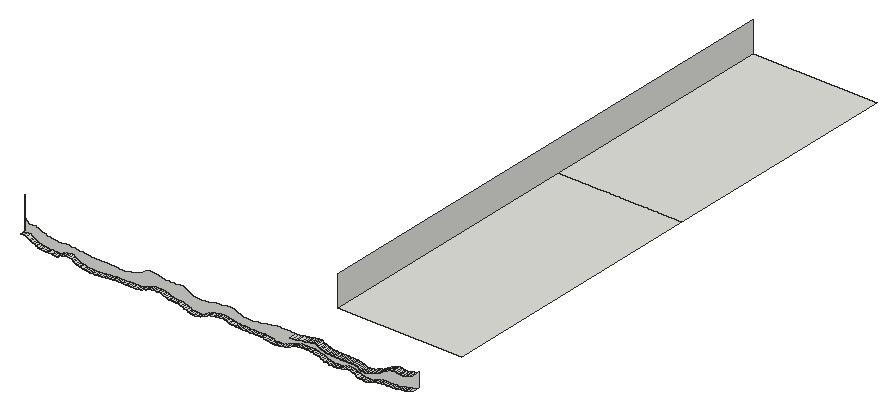
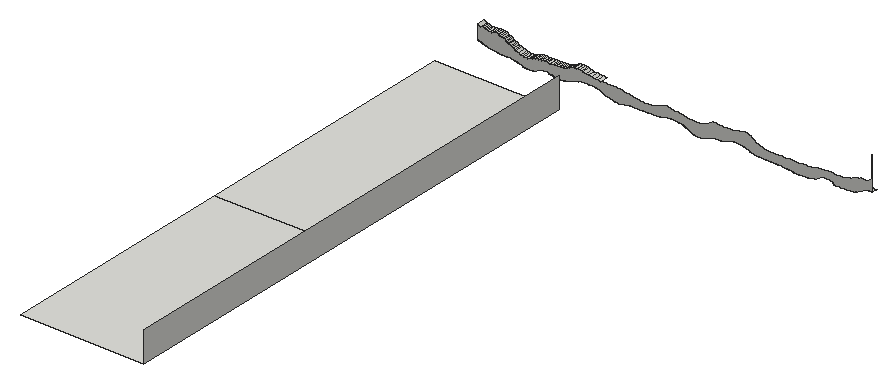
# SketchUp Ruby script. Lengths in inches.
U = 1.inch
M = Sketchup.active_model
def pt(a) = Geom::Point3d.new(a.map { |v| v * U })
def face(e, loops, mat)
  f = e.add_face(loops[0].map { |a| pt(a) })
  loops[1..].each { |l| e.add_face(l.map { |a| pt(a) }).erase! }
  f.material = f.back_material = mat if mat
  f
end
# faces: each face lists its corners as indices into pts; further lists are holes
def faces(e, pts, list, mat = nil) = list.each { |f| face(e, (f[0].is_a?(Array) ? f : [f]).map { |l| l.map { |i| pts[i] } }, mat) }
# xy, xz, yz: faces in a plane at the given z, y or x. An outline is a flat list of corners, or four numbers for a rectangle; further outlines are holes
def ring(l) = l.size == 4 ? [[l[0], l[1]], [l[2], l[1]], [l[2], l[3]], [l[0], l[3]]] : l.each_slice(2).to_a
def flat(e, list, mat, &to3) = list.each { |f| face(e, (f[0].is_a?(Array) ? f : [f]).map { |l| ring(l).map { |u, v| to3.(u, v) } }, mat) }
def xy(e, z, list, mat = nil) = flat(e, list, mat) { |x, y| [x, y, z] }
def xz(e, y, list, mat = nil) = flat(e, list, mat) { |x, z| [x, y, z] }
def yz(e, x, list, mat = nil) = flat(e, list, mat) { |y, z| [x, y, z] }
def lines(e, pts, list) = list.each { |a, b| e.add_line(pt(pts[a]), pt(pts[b])) }
# prism: a flat outline (further loops are holes) pulled along v
def prism(e, loops, v, mat = nil)
  f = face(e, loops, mat); d = Geom::Vector3d.new(v.map { |x| x * U })
  f.pushpull(f.normal.samedirection?(d) ? d.length : -d.length)
end
def box(e, o, s, mat = nil) = prism(e, [[o, [o[0] + s[0], o[1], o[2]], [o[0] + s[0], o[1] + s[1], o[2]], [o[0], o[1] + s[1], o[2]]]], [0, 0, s[2]], mat)
def at(x, y, z, deg = 0) = Geom::Transformation.translation(pt([x, y, z])) * Geom::Transformation.rotation(ORIGIN, Z_AXIS, deg.degrees)
def axes(o, x, y, z) = Geom::Transformation.new([*x, 0, *y, 0, *z, 0, *pt(o).to_a, 1])
def part(name) = M.definitions.add(name)
# library, detail: a bought-in or finely detailed component or shape, given as its bounding box
def library(name, o, s) = part(name).tap { |d| box(d.entities, o, s) }
def detail(e, o, s) = box(e.add_group.entities, o, s)
def put(e, d, t, mat = nil) = e.add_instance(d, t).tap { |i| i.material = mat if mat }
def group(e, t, mat = nil) = e.add_group.tap { |g| g.transformation = t; g.material = mat if mat }.entities
root = M.entities
xy(root,237.65,[[2918.33,566.68,2919.02,568.68],[2919.02,566.68,2919.64,568.68]])
xy(root,238.18,[[3012.28,566.68,3012.96,568.68]])
xy(root,238.33,[[2927.43,566.68,2927.98,568.68],[2927.98,566.68,2928.66,568.68]])
xy(root,238.34,[[2929.34,566.68,2930.27,568.68],[2930.27,566.68,2930.76,568.68],[2930.76,566.68,2931.52,568.68],[2931.52,566.68,2932.15,568.68],[2932.15,566.68,2932.9,568.68],
  [2932.9,566.68,2933.52,568.68],[2933.52,566.68,2934.29,568.68],[2934.29,566.68,2934.91,568.68]])
xy(root,238.62,[[2978.81,566.68,2979.58,568.68],[2979.58,566.68,2980.21,568.68],[2980.21,566.68,2980.97,568.68],[2980.97,566.68,2981.59,568.68],[2981.59,566.68,2982.44,568.68],
  [2982.44,566.68,2983.08,568.68],[2983.08,566.68,2983.7,568.68]])
xy(root,238.625,[[2977.39,566.68,2978.25,568.68]])
xy(root,238.89,[[3033.2,566.68,3033.88,568.68]])
xy(root,238.9,[[3034.64,566.68,3035.26,568.68],[3035.26,566.68,3036.03,568.68]])
xy(root,240.43,[[3001.48,566.68,3002.05,568.68]])
xy(root,241.52,[[2889.03,566.68,2889.09,568.68]])
xy(root,242.28,[[3019.3,565.74,3019.8125,568.68]])
xy(root,242.3,[[3017.54,565.74,3018.21,568.68]])
xy(root,242.33,[[3015.13,565.74,3015.71,568.68]])
xy(root,242.625,[[2994.64,589.83,3043.1,697.21],[2994.64,697.21,3043.1,792.52]])
xz(root,568.68,[[2957.95,236.98,2957.34,237.01,2956.65,237.04,2955.89,237.11,2955.2,237.2,2954.67,237.33,2954,237.68,2953.0625,237.96,2952.5,238.28,2951.72,238.43,2950.94,238.78,2950.27,238.79,2949.73,238.8,2948.97,238.83,2948.22,238.875,2947.65,238.94,2947.07,239.04,2946.41,239.29,2945.83,239.53,2945.3,239.7,2944.61,239.92,2943.98,240.11,2943.2,240.27,2942.58,240.25,2941.875,240.23,2941.11,240.19,2940.4375,240.12,2939.78,240.03,2939.14,239.85,2938.59,239.52,2938.03,239.35,2937.44,239.18,2936.93,238.86,2936.24,238.72,2935.42,238.59,2934.91,238.34,2929.34,238.34,2928.66,238.33,2927.43,238.33,2926.71,238.32,2925.86,238.3,2925.23,238.28,2924.48,238.26,2923.85,238.15,2923.09,238.13,2922.54,238.1,2921.6875,237.98,2921.07,237.94,2920.31,237.89,2919.64,237.65,2918.33,237.65,2917.64,237.66,2916.89,237.67,2916.29,237.68,2915.68,237.71,2914.97,237.76,2914.28,237.82,2913.62,237.9,2912.68,238.21,2912.21,238.31,2911.3,238.43,2910.65,238.74,2910.07,239.11,2909.49,239.38,2909.03,239.71,2908.33,240.11,2907.64,240.09,2906.98,240.05,2906.39,239.99,2905.66,239.88,2905.11,239.69,2904.53,239.55,2903.97,238.9375,2903.44,238.77,2902.7,238.79,2901.83,238.8,2901.32,238.82,2900.28,238.92,2899.59,238.93,2898.89,238.94,2898.19,238.97,2897.51,239.03,2896.82,239.09,2896.04,239.19,2895.53,239.52,2894.97,239.64,2894.52,239.86,2893.73,240.2,2893.13,240.59,2892.59,240.85,2891.57,241.55,2890.3,241.69,2889.09,241.52,2889.09,246.2,2890.66,244.96,2892.05,244.9375,2893.3,244.92,2893.52,244.61,2894.08,244.54,2894.84,244.41,2895.51,244.11,2896.03,243.95,2896.69,243.79,2897.21,243.48,2897.85,243.3,2898.4375,243.14,2898.92,243.06,2899.64,242.85,2900.22,242.78,2901.03,242.73,2901.57,242.68,2902.24,242.51,2902.76,242.46,2903.3,242.58,2903.93,242.57,2904.56,242.81,2905.13,242.86,2905.69,242.89,2906.33,242.92,2906.76,242.625,2907.37,242.65,2907.92,242.62,2908.55,242.58,2909.11,242.57,2909.75,242.48,2910.41,242.38,2911.07,242.34,2911.74,242.24,2912.91,241.96,2913.68,241.89,2914.5,241.83,2915.1,241.78,2915.87,241.75,2916.32,241.74,2916.87,241.72,2918.13,241.7,2918.86,241.69,2919.53,241.68,2920.12,241.68,2920.61,241.67,2921.3125,241.74,2921.88,241.75,2923.88,241.75,2924.37,241.67,2924.9,241.66,2925.51,241.57,2926.05,241.53,2926.67,241.51,2927.22,241.49,2927.92,241.48,2928.58,241.47,2929.15,241.46,2929.86,241.6,2930.59,241.85,2931.26,241.91,2932.16,242.1,2932.93,242.46,2933.63,242.78,2934.4,242.97,2934.93,243.23,2935.33,243.48,2935.85,243.72,2936.1875,244.12,2936.66,244.39,2937.14,244.73,2937.625,244.87,2938.21,244.95,2938.89,245.01,2939.54,244.81,2940.11,244.7,2940.59,244.67,2941.2,244.55,2941.74,244.51,2942.2,244.25,2942.95,244.11,2943.51,244.04,2944.13,243.99,2944.85,243.95,2945.35,243.93,2946.04,243.91,2946.61,243.89,2947.31,243.88,2947.96,243.94,2948.6,243.95,2949.16,244.1,2949.79,244.13,2950.27,244.15,2950.79,244.17,2951.31,244.18,2951.91,243.8,2952.45,243.43,2953.06,243.09,2953.45,242.875,2953.95,242.68,2954.54,242.51,2955.05,242.21,2955.65,242.11,2956.33,241.96,2956.89,241.89,2957.35,241.85,2957.87,241.8125,2958.38,241.79,2958.96,241.78,2959.63,241.91,2960.1,241.93,2960.77,242.09,2961.54,242.2,2962.04,242.24,2962.65,242.42,2963.2,242.47,2963.95,242.71,2964.59,242.78,2965.07,242.82,2965.76,242.85,2966.46,242.87,2967.01,243.02,2967.63,243.05,2968.18,243.29,2968.86,243.35,2969.41,243.39,2970.01,243.42,2970.78,243.14,2971.35,242.9375,2971.9,242.65,2972.52,242.39,2973.28,242.14,2973.92,241.89,2974.41,241.78,2975.46,241.63,2976.23,241.56,2976.83,241.51,2977.28,241.48,2977.8,241.46,2978.67,241.51,2979.39,241.59,2980.33,241.82,2981.11,241.87,2981.875,241.98,2982.49,242.02,2983.14,242.19,2983.84,242.38,2984.33,242.4375,2984.85,242.48,2985.51,242.58,2986.04,242.61,2986.625,242.77,2987.08,242.95,2987.64,243.01,2988.15,243.05,2988.72,243.08,2989.375,243.09,2991.53,243.09,2992.1,243.08,2992.6875,243.07,2993.27,243.07,2993.93,243.0625,2994.54,243.05,2995.22,243.05,2996.49,243.1,2997.66,243.17,2998.8,243.4,3000.0625,243.52,3001.19,243.71,3002.09,243.99,3002.79,244.08,3003.49,244.21,3004.07,244.27,3004.61,244.3,3005.28,244.39,3005.875,244.19,3006.25,243.88,3006.73,243.59,3007.28,243.33,3007.83,243.22,3008.32,242.92,3008.8,242.75,3009.36,242.6,3009.92,242.52,3010.48,242.47,3011.0625,242.43,3011.64,242.4,3012.22,242.39,3012.8,242.37,3013.38,242.36,3013.97,242.35,3015.13,242.33,3015.71,242.33,3016.43,242.32,3016.9,242.3125,3017.54,242.3,3018.21,242.3,3018.66,242.29,3019.3,242.28,3019.8125,242.28,3020.44,242.2,3021.02,241.97,3021.59,241.84,3022.1,241.57,3022.52,241.33,3022.99,241.24,3023.52,241.17,3023.99,241.12,3024.59,241.09,3025.16,241.14,3025.8,241.35,3026.39,241.46,3027.33,241.85,3028.33,242.23,3028.89,242.42,3029.61,242.61,3030.125,242.91,3030.5,243.14,3031.04,243.52,3031.52,243.71,3031.85,244.02,3032.29,244.21,3032.88,244.57,3033.35,244.76,3033.97,245.125,3034.47,245.32,3034.95,245.41,3035.5,245.48,3035.99,245.59,3036.52,245.55,3037.13,245.35,3037.62,245.31,3038.17,245.27,3038.73,245.24,3039.29,245.22,3039.85,245.34,3040.48,245.42,3041.0625,245.52,3041.44,245.76,3041.91,245.9,3043.1,246.43,3043.1,240.89,3041.27,240.1,3040.71,239.96,3040.1875,239.81,3039.5,239.53,3038.95,239.49,3038.23,239.42,3037.43,239.28,3036.66,239.15,3036.03,238.9,3034.64,238.9,3033.88,238.89,3033.2,238.89,3032.52,238.88,3031.98,238.875,3031.22,238.86,3030.48,238.83,3029.91,238.8,3029.33,238.74,3028.67,238.6,3028.1,238.51,3027.57,238.33,3026.88,238.08,3026.2,237.84,3025.51,237.5625,3024.91,237.47,3024.23,237.4,3023.5,237.42,3022.93,237.45,3022.34,237.51,3021.74,237.59,3021.2,237.71,3020.37,238,3019.66,238.33,3019.11,238.57,3018.61,238.86,3018.09,238.96,3017.4,239.02,3016.72,239.125,3015.98,239.04,3015.41,238.66,3014.82,238.61,3014.16,238.55,3013.64,238.27,3012.96,238.18,3012.28,238.18,3011.61,238.11,3011.08,238.15,3010.26,238.19,3009.6875,238.26,3009.12,238.48,3008.46,238.56,3007.89,238.67,3007.37,239.01,3006.6875,239.18,3006.0625,239.5,3005.3,239.65,3004.6875,239.8,3003.93,239.96,3003.28,240.23,3002.7,240.27,3002.05,240.43,3001.48,240.43,3000.9,240.42,3000.375,240.41,2999.68,240.4,2998.99,240.37,2998.3,240.33,2997.62,240.27,2996.94,240.17,2996.32,239.97,2995.67,239.75,2994.93,239.375,2994.14,239.08,2993.26,238.72,2992.51,238.46,2991.29,238.14,2990.17,237.88,2989.52,237.87,2988.65,237.74,2987.94,237.79,2987.17,237.86,2986.54,238.15,2985.77,238.19,2985.15,238.25,2984.39,238.45,2983.7,238.62,2978.81,238.62,2978.25,238.625,2977.39,238.625,2976.7,238.63,2976.08,238.64,2975.3,238.65,2974.63,238.66,2973.94,238.6875,2973.27,238.73,2972.79,238.78,2971.91,238.93,2971.14,239.07,2970.59,239.16,2969.74,239.44,2969.07,239.56,2968.46,239.72,2967.73,239.7,2967.17,239.69,2966.58,239.65,2965.96,239.6,2965.47,239.54,2964.66,239.31,2963.66,239.22,2963.08,239.12,2962.4375,238.76,2961.8,238.51,2961.24,238.375,2960.8,238.02,2960.1,237.74,2959.48,237.43,2958.63,237.22],[2889.03,241.52,2889.09,254.5]])
yz(root,2994.64,[[589.83,242.625,792.52,254.5]])
p = [[2955.89,568.68,237.11],[2956.65,568.68,237.04],[2956.65,566.68,237.04],[2955.89,566.68,237.11],[2957.34,568.68,237.01],[2957.34,566.68,237.01],
  [2957.95,568.68,236.98],[2957.95,566.68,236.98],[2958.63,568.68,237.22],[2958.63,566.68,237.22],[2955.2,568.68,237.2],[2955.2,566.68,237.2],
  [2954.67,568.68,237.33],[2954.67,566.68,237.33],[2959.48,568.68,237.43],[2959.48,566.68,237.43],[2954,568.68,237.68],[2954,566.68,237.68],
  [2960.1,568.68,237.74],[2960.1,566.68,237.74],[3022.93,568.68,237.45],[3023.5,568.68,237.42],[3023.5,566.68,237.42],[3022.93,566.68,237.45],
  [3024.23,568.68,237.4],[3024.23,566.68,237.4],[3024.91,568.68,237.47],[3024.91,566.68,237.47],[3021.74,568.68,237.59],[3022.34,568.68,237.51],
  [3022.34,566.68,237.51],[3021.74,566.68,237.59],[3025.51,568.68,237.5625],[3025.51,566.68,237.5625],[2919.64,568.68,237.65],[2920.31,568.68,237.89],
  [2920.31,566.68,237.89],[2919.64,566.68,237.65],[3021.2,568.68,237.71],[3021.2,566.68,237.71],[3026.2,568.68,237.84],[3026.2,566.68,237.84],
  [2914.97,568.68,237.76],[2915.68,568.68,237.71],[2915.68,566.68,237.71],[2914.97,566.68,237.76],[2916.29,568.68,237.68],[2916.29,566.68,237.68],
  [2916.89,568.68,237.67],[2916.89,566.68,237.67],[2917.64,568.68,237.66],[2917.64,566.68,237.66],[2918.33,568.68,237.65],[2918.33,566.68,237.65],
  [2953.0625,568.68,237.96],[2953.0625,566.68,237.96],[2960.8,568.68,238.02],[2960.8,566.68,238.02],[2987.94,568.68,237.79],[2988.65,568.68,237.74],
  [2988.65,566.68,237.74],[2987.94,566.68,237.79],[2989.52,568.68,237.87],[2989.52,566.68,237.87],[3020.37,568.68,238],[3020.37,566.68,238],
  [2913.62,568.68,237.9],[2914.28,568.68,237.82],[2914.28,566.68,237.82],[2913.62,566.68,237.9],[2987.17,568.68,237.86],[2987.17,566.68,237.86],
  [3026.88,568.68,238.08],[3026.88,566.68,238.08],[2912.68,568.68,238.21],[2912.68,566.68,238.21],[2921.07,568.68,237.94],[2921.07,566.68,237.94],
  [2921.6875,568.68,237.98],[2921.6875,566.68,237.98],[2986.54,568.68,238.15],[2986.54,566.68,238.15],[2990.17,568.68,237.88],[2990.17,566.68,237.88],
  [2991.29,568.68,238.14],[2991.29,566.68,238.14],[2922.54,568.68,238.1],[2922.54,566.68,238.1],[2952.5,568.68,238.28],[2952.5,566.68,238.28],
  [2961.24,568.68,238.375],[2961.24,566.68,238.375],[3019.66,568.68,238.33],[3019.66,566.68,238.33],[2923.09,568.68,238.13],[2923.09,566.68,238.13],
  [2923.85,568.68,238.15],[2923.85,566.68,238.15],[2985.77,568.68,238.19],[2985.77,566.68,238.19],[2992.51,568.68,238.46],[2992.51,566.68,238.46],
  [3010.26,568.68,238.19],[3011.08,568.68,238.15],[3011.08,566.68,238.15],[3010.26,566.68,238.19],[3011.61,568.68,238.11],[3011.61,566.68,238.11],
  [3012.28,568.68,238.18],[3012.28,566.68,238.18],[3027.57,568.68,238.33],[3027.57,566.68,238.33],[2912.21,568.68,238.31],[2912.21,566.68,238.31],
  [2924.48,568.68,238.26],[2924.48,566.68,238.26],[2985.15,568.68,238.25],[2985.15,566.68,238.25],[3009.6875,568.68,238.26],[3009.6875,566.68,238.26],
  [3012.96,568.68,238.18],[3013.64,568.68,238.27],[3013.64,566.68,238.27],[3012.96,566.68,238.18],[2911.3,568.68,238.43],[2911.3,566.68,238.43],
  [2925.23,568.68,238.28],[2925.23,566.68,238.28],[2925.86,568.68,238.3],[2925.86,566.68,238.3],[2926.71,568.68,238.32],[2926.71,566.68,238.32],
  [2927.43,568.68,238.33],[2927.43,566.68,238.33],[2928.66,568.68,238.33],[2929.34,568.68,238.34],[2929.34,566.68,238.34],[2928.66,566.68,238.33],
  [2934.91,568.68,238.34],[2935.42,568.68,238.59],[2935.42,566.68,238.59],[2934.91,566.68,238.34],[2951.72,568.68,238.43],[2951.72,566.68,238.43],
  [2984.39,568.68,238.45],[2984.39,566.68,238.45],[3009.12,568.68,238.48],[3009.12,566.68,238.48],[3014.16,568.68,238.55],[3014.16,566.68,238.55],
  [3019.11,568.68,238.57],[3019.11,566.68,238.57],[3028.1,568.68,238.51],[3028.1,566.68,238.51],[2910.65,568.68,238.74],[2910.65,566.68,238.74],
  [2950.94,568.68,238.78],[2950.94,566.68,238.78],[2961.8,568.68,238.51],[2961.8,566.68,238.51],[2962.4375,568.68,238.76],[2962.4375,566.68,238.76],
  [2983.7,568.68,238.62],[2983.7,566.68,238.62],[2993.26,568.68,238.72],[2993.26,566.68,238.72],[3008.46,568.68,238.56],[3008.46,566.68,238.56],
  [3014.82,568.68,238.61],[3014.82,566.68,238.61],[3028.67,568.68,238.6],[3028.67,566.68,238.6],[2936.24,568.68,238.72],[2936.24,566.68,238.72],
  [2974.63,568.68,238.66],[2975.3,568.68,238.65],[2975.3,566.68,238.65],[2974.63,566.68,238.66],[2976.08,568.68,238.64],[2976.08,566.68,238.64],
  [2976.7,568.68,238.63],[2976.7,566.68,238.63],[2977.39,568.68,238.625],[2977.39,566.68,238.625],[2978.25,568.68,238.625],[2978.81,568.68,238.62],
  [2978.81,566.68,238.62],[2978.25,566.68,238.625],[3007.89,568.68,238.67],[3007.89,566.68,238.67],[3015.41,568.68,238.66],[3015.41,566.68,238.66],
  [3018.61,568.68,238.86],[3018.61,566.68,238.86],[3029.33,568.68,238.74],[3029.33,566.68,238.74],[2910.07,568.68,239.11],[2910.07,566.68,239.11],
  [2936.93,568.68,238.86],[2936.93,566.68,238.86],[2972.79,568.68,238.78],[2973.27,568.68,238.73],[2973.27,566.68,238.73],[2972.79,566.68,238.78],
  [2973.94,568.68,238.6875],[2973.94,566.68,238.6875],[2994.14,568.68,239.08],[2994.14,566.68,239.08],[3007.37,568.68,239.01],[3007.37,566.68,239.01],
  [3015.98,568.68,239.04],[3015.98,566.68,239.04],[3029.91,568.68,238.8],[3029.91,566.68,238.8],[2900.28,568.68,238.92],[2901.32,568.68,238.82],
  [2901.32,566.68,238.82],[2900.28,566.68,238.92],[2901.83,568.68,238.8],[2901.83,566.68,238.8],[2902.7,568.68,238.79],[2902.7,566.68,238.79],
  [2903.44,568.68,238.77],[2903.44,566.68,238.77],[2903.97,568.68,238.9375],[2903.97,566.68,238.9375],[2948.22,568.68,238.875],[2948.97,568.68,238.83],
  [2948.97,566.68,238.83],[2948.22,566.68,238.875],[2949.73,568.68,238.8],[2949.73,566.68,238.8],[2950.27,568.68,238.79],[2950.27,566.68,238.79],
  [2963.08,568.68,239.12],[2963.08,566.68,239.12],[2971.91,568.68,238.93],[2971.91,566.68,238.93],[3030.48,568.68,238.83],[3030.48,566.68,238.83],
  [3031.22,568.68,238.86],[3031.22,566.68,238.86],[2898.19,568.68,238.97],[2898.89,568.68,238.94],[2898.89,566.68,238.94],[2898.19,566.68,238.97],
  [2899.59,568.68,238.93],[2899.59,566.68,238.93],[2904.53,568.68,239.55],[2904.53,566.68,239.55],[2937.44,568.68,239.18],[2937.44,566.68,239.18],
  [2947.07,568.68,239.04],[2947.65,568.68,238.94],[2947.65,566.68,238.94],[2947.07,566.68,239.04],[2971.14,568.68,239.07],[2971.14,566.68,239.07],
  [3018.09,568.68,238.96],[3018.09,566.68,238.96],[3031.98,568.68,238.875],[3031.98,566.68,238.875],[3032.52,568.68,238.88],[3032.52,566.68,238.88],
  [3033.2,568.68,238.89],[3033.2,566.68,238.89],[3033.88,568.68,238.89],[3034.64,568.68,238.9],[3034.64,566.68,238.9],[3033.88,566.68,238.89],
  [3036.03,568.68,238.9],[3036.66,568.68,239.15],[3036.66,566.68,239.15],[3036.03,566.68,238.9],[2896.82,568.68,239.09],[2897.51,568.68,239.03],
  [2897.51,566.68,239.03],[2896.82,566.68,239.09],[2946.41,568.68,239.29],[2946.41,566.68,239.29],[3006.6875,568.68,239.18],[3006.6875,566.68,239.18],
  [3016.72,568.68,239.125],[3016.72,566.68,239.125],[3017.4,568.68,239.02],[3017.4,566.68,239.02],[2896.04,568.68,239.19],[2896.04,566.68,239.19],
  [2909.49,568.68,239.38],[2909.49,566.68,239.38],[2963.66,568.68,239.22],[2963.66,566.68,239.22],[2970.59,568.68,239.16],[2970.59,566.68,239.16],
  [2994.93,568.68,239.375],[2994.93,566.68,239.375],[2895.53,568.68,239.52],[2895.53,566.68,239.52],[2938.03,568.68,239.35],[2938.03,566.68,239.35],
  [2964.66,568.68,239.31],[2964.66,566.68,239.31],[2969.74,568.68,239.44],[2969.74,566.68,239.44],[3006.0625,568.68,239.5],[3006.0625,566.68,239.5],
  [3037.43,568.68,239.28],[3037.43,566.68,239.28],[2945.83,568.68,239.53],[2945.83,566.68,239.53],[2965.47,568.68,239.54],[2965.47,566.68,239.54],
  [3038.23,568.68,239.42],[3038.23,566.68,239.42],[2909.03,568.68,239.71],[2909.03,566.68,239.71],[2938.59,568.68,239.52],[2938.59,566.68,239.52],
  [2969.07,568.68,239.56],[2969.07,566.68,239.56],[2995.67,568.68,239.75],[2995.67,566.68,239.75],[3038.95,568.68,239.49],[3038.95,566.68,239.49],
  [2894.97,568.68,239.64],[2894.97,566.68,239.64],[2939.14,568.68,239.85],[2939.14,566.68,239.85],[2945.3,568.68,239.7],[2945.3,566.68,239.7],
  [2965.96,568.68,239.6],[2965.96,566.68,239.6],[3005.3,568.68,239.65],[3005.3,566.68,239.65],[3039.5,568.68,239.53],[3039.5,566.68,239.53],
  [3040.1875,568.68,239.81],[3040.1875,566.68,239.81],[2894.52,568.68,239.86],[2894.52,566.68,239.86],[2905.11,568.68,239.69],[2905.11,566.68,239.69],
  [2966.58,568.68,239.65],[2966.58,566.68,239.65],[2967.17,568.68,239.69],[2967.17,566.68,239.69],[2968.46,568.68,239.72],[2968.46,566.68,239.72],
  [2905.66,568.68,239.88],[2905.66,566.68,239.88],[2908.33,568.68,240.11],[2908.33,566.68,240.11],[2944.61,568.68,239.92],[2944.61,566.68,239.92],
  [2967.73,568.68,239.7],[2967.73,566.68,239.7],[2996.32,568.68,239.97],[2996.32,566.68,239.97],[3004.6875,568.68,239.8],[3004.6875,566.68,239.8],
  [2939.78,568.68,240.03],[2939.78,566.68,240.03],[3003.93,568.68,239.96],[3003.93,566.68,239.96],[3040.71,568.68,239.96],[3040.71,566.68,239.96],
  [2893.73,568.68,240.2],[2893.73,566.68,240.2],[2906.39,568.68,239.99],[2906.39,566.68,239.99],[2943.98,568.68,240.11],[2943.98,566.68,240.11],
  [2906.98,568.68,240.05],[2906.98,566.68,240.05],[2907.64,568.68,240.09],[2907.64,566.68,240.09],[2940.4375,568.68,240.12],[2940.4375,566.68,240.12],
  [2996.94,568.68,240.17],[2996.94,566.68,240.17],[3003.28,568.68,240.23],[3003.28,566.68,240.23],[3041.27,568.68,240.1],[3041.27,566.68,240.1],
  [2941.11,568.68,240.19],[2941.11,566.68,240.19],[2943.2,568.68,240.27],[2943.2,566.68,240.27],[3043.1,568.68,240.89],[3043.1,566.68,240.89],
  [2893.13,568.68,240.59],[2893.13,566.68,240.59],[2941.875,568.68,240.23],[2941.875,566.68,240.23],[2942.58,568.68,240.25],[2942.58,566.68,240.25],
  [2997.62,568.68,240.27],[2997.62,566.68,240.27],[3002.7,568.68,240.27],[3002.7,566.68,240.27],[2998.3,568.68,240.33],[2998.3,566.68,240.33],
  [2998.99,568.68,240.37],[2998.99,566.68,240.37],[3002.05,568.68,240.43],[3002.05,566.68,240.43],[2999.68,568.68,240.4],[2999.68,566.68,240.4],
  [3000.375,568.68,240.41],[3000.375,566.68,240.41],[3000.9,568.68,240.42],[3000.9,566.68,240.42],[3001.48,568.68,240.43],[3001.48,566.68,240.43],
  [2892.59,568.68,240.85],[2892.59,566.68,240.85],[2891.57,568.68,241.55],[2891.57,566.68,241.55],[3023.52,568.68,241.17],[3023.99,568.68,241.12],
  [3023.99,565.74,241.12],[3023.52,565.74,241.17],[3024.59,568.68,241.09],[3024.59,565.74,241.09],[3025.16,568.68,241.14],[3025.16,565.74,241.14],
  [3025.8,568.68,241.35],[3025.8,565.74,241.35],[3022.52,568.68,241.33],[3022.99,568.68,241.24],[3022.99,565.74,241.24],[3022.52,565.74,241.33],
  [3022.1,568.68,241.57],[3022.1,565.74,241.57],[3026.39,568.68,241.46],[3026.39,565.74,241.46],[3027.33,568.68,241.85],[3027.33,565.74,241.85],
  [2889.09,568.68,241.52],[2890.3,568.68,241.69],[2890.3,566.68,241.69],[2889.09,566.68,241.52],[3021.59,568.68,241.84],[3021.59,565.74,241.84],
  [3021.02,568.68,241.97],[3021.02,565.74,241.97],[3028.33,568.68,242.23],[3028.33,565.74,242.23],[3020.44,568.68,242.2],[3020.44,565.74,242.2],
  [3019.8125,568.68,242.28],[3019.8125,565.74,242.28],[3028.89,568.68,242.42],[3028.89,565.74,242.42],[3013.97,568.68,242.35],[3014.55,568.68,242.34],
  [3014.55,565.74,242.34],[3013.97,565.74,242.35],[3015.13,568.68,242.33],[3015.13,565.74,242.33],[3015.71,568.68,242.33],[3016.43,568.68,242.32],
  [3016.43,565.74,242.32],[3015.71,565.74,242.33],[3016.9,568.68,242.3125],[3016.9,565.74,242.3125],[3017.54,568.68,242.3],[3017.54,565.74,242.3],
  [3018.21,568.68,242.3],[3018.66,568.68,242.29],[3018.66,565.74,242.29],[3018.21,565.74,242.3],[3019.3,568.68,242.28],[3019.3,565.74,242.28],
  [3010.48,568.68,242.47],[3011.0625,568.68,242.43],[3011.0625,565.74,242.43],[3010.48,565.74,242.47],[3011.64,568.68,242.4],[3011.64,565.74,242.4],
  [3012.22,568.68,242.39],[3012.22,565.74,242.39],[3012.8,568.68,242.37],[3012.8,565.74,242.37],[3013.38,568.68,242.36],[3013.38,565.74,242.36],
  [3029.61,568.68,242.61],[3029.61,565.74,242.61],[3009.36,568.68,242.6],[3009.92,568.68,242.52],[3009.92,565.74,242.52],[3009.36,565.74,242.6],
  [3008.8,568.68,242.75],[3008.8,565.74,242.75],[3030.125,568.68,242.91],[3030.125,565.74,242.91],[3008.32,568.68,242.92],[3008.32,565.74,242.92],
  [3007.83,568.68,243.22],[3007.83,565.74,243.22],[3030.5,568.68,243.14],[3030.5,565.74,243.14],[2995.22,568.68,243.05],[2996.49,568.68,243.1],
  [2996.49,565.74,243.1],[2995.22,565.74,243.05],[2997.66,568.68,243.17],[2997.66,565.74,243.17],[3031.04,568.68,243.52],[3031.04,565.74,243.52],
  [2998.8,568.68,243.4],[2998.8,565.74,243.4],[3007.28,568.68,243.33],[3007.28,565.74,243.33],[3006.73,568.68,243.59],[3006.73,565.74,243.59],
  [3000.0625,568.68,243.52],[3000.0625,565.74,243.52],[3001.19,568.68,243.71],[3001.19,565.74,243.71],[3031.52,568.68,243.71],[3031.52,565.74,243.71],
  [3006.25,568.68,243.88],[3006.25,565.74,243.88],[3002.09,568.68,243.99],[3002.09,565.74,243.99],[3031.85,568.68,244.02],[3031.85,565.74,244.02],
  [3005.875,568.68,244.19],[3005.875,565.74,244.19],[3002.79,568.68,244.08],[3002.79,565.74,244.08],[3032.29,568.68,244.21],[3032.29,565.74,244.21],
  [3003.49,568.68,244.21],[3003.49,565.74,244.21],[3004.07,568.68,244.27],[3004.07,565.74,244.27],[3005.28,568.68,244.39],[3005.28,565.74,244.39],
  [3032.88,568.68,244.57],[3032.88,565.74,244.57],[3004.61,568.68,244.3],[3004.61,565.74,244.3],[3033.35,568.68,244.76],[3033.35,565.74,244.76],
  [3033.97,568.68,245.125],[3033.97,565.74,245.125],[3034.47,568.68,245.32],[3034.47,565.74,245.32],[3038.17,568.68,245.27],[3038.73,568.68,245.24],
  [3038.73,565.74,245.24],[3038.17,565.74,245.27],[3039.29,568.68,245.22],[3039.29,565.74,245.22],[3039.85,568.68,245.34],[3039.85,565.74,245.34],
  [3034.95,568.68,245.41],[3034.95,565.74,245.41],[3036.52,568.68,245.55],[3037.13,568.68,245.35],[3037.13,565.74,245.35],[3036.52,565.74,245.55],
  [3037.62,568.68,245.31],[3037.62,565.74,245.31],[3040.48,568.68,245.42],[3040.48,565.74,245.42],[3035.5,568.68,245.48],[3035.5,565.74,245.48],
  [3041.0625,568.68,245.52],[3041.0625,565.74,245.52],[3035.99,568.68,245.59],[3035.99,565.74,245.59],[3041.44,568.68,245.76],[3041.44,565.74,245.76],
  [3041.91,568.68,245.9],[3041.91,565.74,245.9],[3043.1,568.68,246.43],[3043.1,565.74,246.43]]
faces(root,p,[[0,1,2,3],[1,4,5,2],[4,6,7,5],[6,8,9,7],[10,0,3,11],[12,10,11,13],[8,14,15,9],[16,12,13,17],
  [14,18,19,15],[20,21,22,23],[21,24,25,22],[24,26,27,25],[28,29,30,31],[29,20,23,30],[26,32,33,27],[34,35,36,37],
  [38,28,31,39],[32,40,41,33],[42,43,44,45],[43,46,47,44],[46,48,49,47],[48,50,51,49],[50,52,53,51],[54,16,17,55],
  [18,56,57,19],[58,59,60,61],[59,62,63,60],[64,38,39,65],[66,67,68,69],[67,42,45,68],[70,58,61,71],[40,72,73,41],
  [74,66,69,75],[35,76,77,36],[76,78,79,77],[80,70,71,81],[62,82,83,63],[82,84,85,83],[78,86,87,79],[88,54,55,89],
  [56,90,91,57],[92,64,65,93],[86,94,95,87],[94,96,97,95],[98,80,81,99],[84,100,101,85],[102,103,104,105],[103,106,107,104],
  [106,108,109,107],[72,110,111,73],[112,74,75,113],[96,114,115,97],[116,98,99,117],[118,102,105,119],[120,121,122,123],[124,112,113,125],
  [114,126,127,115],[126,128,129,127],[128,130,131,129],[130,132,133,131],[134,135,136,137],[138,139,140,141],[142,88,89,143],[144,116,117,145],
  [146,118,119,147],[121,148,149,122],[150,92,93,151],[110,152,153,111],[154,124,125,155],[156,142,143,157],[90,158,159,91],[158,160,161,159],
  [162,144,145,163],[100,164,165,101],[166,146,147,167],[148,168,169,149],[152,170,171,153],[139,172,173,140],[174,175,176,177],[175,178,179,176],
  [178,180,181,179],[180,182,183,181],[184,185,186,187],[188,166,167,189],[168,190,191,169],[192,150,151,193],[170,194,195,171],[196,154,155,197],
  [172,198,199,173],[200,201,202,203],[201,204,205,202],[204,174,177,205],[164,206,207,165],[208,188,189,209],[190,210,211,191],[194,212,213,195],
  [214,215,216,217],[215,218,219,216],[218,220,221,219],[220,222,223,221],[222,224,225,223],[226,227,228,229],[227,230,231,228],[230,232,233,231],
  [232,156,157,233],[160,234,235,161],[236,200,203,237],[212,238,239,213],[238,240,241,239],[242,243,244,245],[243,246,247,244],[246,214,217,247],
  [224,248,249,225],[198,250,251,199],[252,253,254,255],[253,226,229,254],[256,236,237,257],[258,192,193,259],[240,260,261,241],[260,262,263,261],
  [262,264,265,263],[266,267,268,269],[270,271,272,273],[274,275,276,277],[275,242,245,276],[278,252,255,279],[280,208,209,281],[210,282,283,211],
  [282,284,285,283],[284,258,259,285],[286,274,277,287],[288,196,197,289],[234,290,291,235],[292,256,257,293],[206,294,295,207],[296,286,287,297],
  [250,298,299,251],[290,300,301,291],[302,292,293,303],[304,280,281,305],[271,306,307,272],[308,278,279,309],[300,310,311,301],[306,312,313,307],
  [314,288,289,315],[298,316,317,299],[318,302,303,319],[294,320,321,295],[312,322,323,313],[324,296,297,325],[316,326,327,317],[328,308,309,329],
  [310,330,331,311],[332,304,305,333],[322,334,335,323],[334,336,337,335],[338,324,325,339],[248,340,341,249],[330,342,343,331],[342,344,345,343],
  [346,318,319,347],[340,348,349,341],[350,314,315,351],[352,328,329,353],[344,354,355,345],[354,346,347,355],[320,356,357,321],[358,332,333,359],
  [326,360,361,327],[362,358,359,363],[336,364,365,337],[366,338,339,367],[348,368,369,349],[370,352,353,371],[368,372,373,369],[372,374,375,373],
  [360,376,377,361],[356,378,379,357],[380,362,363,381],[364,382,383,365],[374,350,351,375],[376,384,385,377],[386,370,371,387],[382,388,389,383],
  [390,366,367,391],[384,392,393,385],[392,394,395,393],[378,396,397,379],[398,380,381,399],[394,386,387,395],[396,400,401,397],[400,402,403,401],
  [404,398,399,405],[402,406,407,403],[406,408,409,407],[408,410,411,409],[410,412,413,411],[414,390,391,415],[416,414,415,417],[418,419,420,421],
  [419,422,423,420],[422,424,425,423],[424,426,427,425],[428,429,430,431],[429,418,421,430],[432,428,431,433],[426,434,435,427],[434,436,437,435],
  [438,439,440,441],[442,432,433,443],[439,416,417,440],[444,442,443,445],[436,446,447,437],[448,444,445,449],[450,448,449,451],[446,452,453,447],
  [454,455,456,457],[455,458,459,456],[460,461,462,463],[461,464,465,462],[464,466,467,465],[468,469,470,471],[469,472,473,470],[474,475,476,477],
  [475,478,479,476],[478,480,481,479],[480,482,483,481],[482,484,485,483],[484,454,457,485],[452,486,487,453],[488,489,490,491],[489,474,477,490],
  [492,488,491,493],[486,494,495,487],[496,492,493,497],[498,496,497,499],[494,500,501,495],[502,503,504,505],[503,506,507,504],[500,508,509,501],
  [506,510,511,507],[512,498,499,513],[514,512,513,515],[510,516,517,511],[516,518,519,517],[508,520,521,509],[522,514,515,523],[518,524,525,519],
  [520,526,527,521],[528,522,523,529],[524,530,531,525],[526,532,533,527],[530,534,535,531],[534,536,537,535],[538,528,529,539],[532,540,541,533],
  [536,542,543,537],[542,538,539,543],[540,544,545,541],[544,546,547,545],[546,548,549,547],[550,551,552,553],[551,554,555,552],[554,556,557,555],
  [548,558,559,549],[560,561,562,563],[561,564,565,562],[564,550,553,565],[556,566,567,557],[558,568,569,559],[566,570,571,567],[568,572,573,569],
  [570,574,575,571],[572,560,563,573],[574,576,577,575],[576,578,579,577]])
